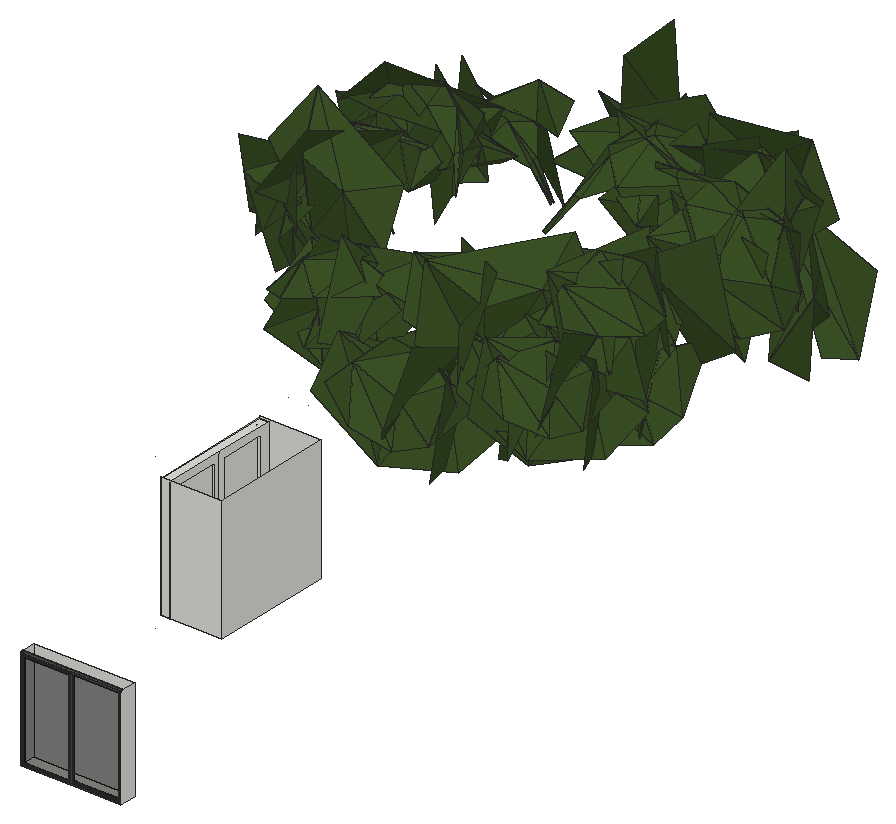
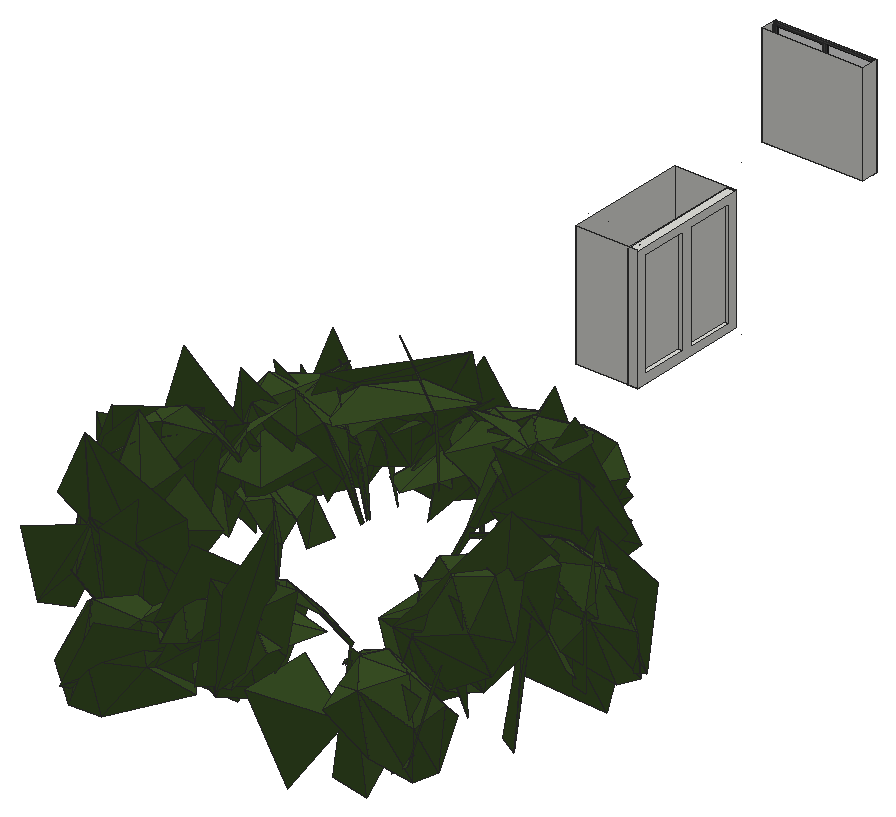
# SketchUp Ruby script. Lengths in inches.
U = 1.inch
M = Sketchup.active_model
def pt(a) = Geom::Point3d.new(a.map { |v| v * U })
def face(e, loops, mat)
  f = e.add_face(loops[0].map { |a| pt(a) })
  loops[1..].each { |l| e.add_face(l.map { |a| pt(a) }).erase! }
  f.material = f.back_material = mat if mat
  f
end
# faces: each face lists its corners as indices into pts; further lists are holes
def faces(e, pts, list, mat = nil) = list.each { |f| face(e, (f[0].is_a?(Array) ? f : [f]).map { |l| l.map { |i| pts[i] } }, mat) }
# xy, xz, yz: faces in a plane at the given z, y or x. An outline is a flat list of corners, or four numbers for a rectangle; further outlines are holes
def ring(l) = l.size == 4 ? [[l[0], l[1]], [l[2], l[1]], [l[2], l[3]], [l[0], l[3]]] : l.each_slice(2).to_a
def flat(e, list, mat, &to3) = list.each { |f| face(e, (f[0].is_a?(Array) ? f : [f]).map { |l| ring(l).map { |u, v| to3.(u, v) } }, mat) }
def xy(e, z, list, mat = nil) = flat(e, list, mat) { |x, y| [x, y, z] }
def xz(e, y, list, mat = nil) = flat(e, list, mat) { |x, z| [x, y, z] }
def yz(e, x, list, mat = nil) = flat(e, list, mat) { |y, z| [x, y, z] }
def lines(e, pts, list) = list.each { |a, b| e.add_line(pt(pts[a]), pt(pts[b])) }
# prism: a flat outline (further loops are holes) pulled along v
def prism(e, loops, v, mat = nil)
  f = face(e, loops, mat); d = Geom::Vector3d.new(v.map { |x| x * U })
  f.pushpull(f.normal.samedirection?(d) ? d.length : -d.length)
end
def box(e, o, s, mat = nil) = prism(e, [[o, [o[0] + s[0], o[1], o[2]], [o[0] + s[0], o[1] + s[1], o[2]], [o[0], o[1] + s[1], o[2]]]], [0, 0, s[2]], mat)
def at(x, y, z, deg = 0) = Geom::Transformation.translation(pt([x, y, z])) * Geom::Transformation.rotation(ORIGIN, Z_AXIS, deg.degrees)
def axes(o, x, y, z) = Geom::Transformation.new([*x, 0, *y, 0, *z, 0, *pt(o).to_a, 1])
def part(name) = M.definitions.add(name)
# library, detail: a bought-in or finely detailed component or shape, given as its bounding box
def library(name, o, s) = part(name).tap { |d| box(d.entities, o, s) }
def detail(e, o, s) = box(e.add_group.entities, o, s)
def put(e, d, t, mat = nil) = e.add_instance(d, t).tap { |i| i.material = mat if mat }
def group(e, t, mat = nil) = e.add_group.tap { |g| g.transformation = t; g.material = mat if mat }.entities
root = M.entities
M.materials.add("AM113_062_Tilia").color = [58, 81, 37]
M.materials.add("Glass_Tinted_Gray").color = [0, 0, 0]
M.materials["Glass_Tinted_Gray"].alpha = 0.125
M.materials.add("[0135_DarkGray]").color = [81, 81, 81]
M.materials.add("[Mirror 02]").color = [229, 229, 229]
M.materials.add("[Terrazzo Light Blue]").color = [196, 214, 227]
c1 = part("Window (2)")
xy(c1.entities,31.72,[[-0.78,88.6,2.72,128.1]])
xy(c1.entities,34.95,[[-0.78,91.53,0.84,106.59],[0.84,91.53,1.05,97.58],[1.05,91.53,1.42,106.59],[1.42,91.53,2.72,106.59],[0.84,97.58,1.05,98.18],
  [0.84,98.18,1.05,106.59]])
xy(c1.entities,35.27,[[-0.78,110.09,0.97,125.14],[1.05,110.09,2.72,125.14]])
xy(c1.entities,58.35,[[2.72,108.74,3.8,109.74]])
xy(c1.entities,77.8125,[[-0.78,110.09,2.72,125.14],[0.97,110.09,1.05,125.14]])
xy(c1.entities,77.93,[[-0.78,91.53,0.84,106.59],[1.05,91.53,1.42,106.59],[1.42,91.53,2.72,106.59]])
xy(c1.entities,80.72,[[-0.78,88.6,2.72,128.1]])
xz(c1.entities,88.6,[[-0.78,31.72,2.72,80.72]])
xz(c1.entities,91.53,[[-0.78,34.95,0.84,77.93],[1.05,34.95,1.42,77.93],[1.42,34.95,2.72,77.93]])
xz(c1.entities,106.59,[[-0.78,34.95,0.84,77.93],[0.84,34.95,1.05,77.93],[0.84,34.95,2.72,77.93]])
xz(c1.entities,108.74,[[3.8,54.35,4.22,54.6,4.22,59.47,2.72,59.97,2.72,58.35,3.8,58.35]])
xz(c1.entities,109.74,[[3.8,54.35,3.8,58.35,2.72,58.35,2.72,59.97,4.22,59.47,4.22,54.6]])
xz(c1.entities,110.09,[[-0.78,35.27,0.97,77.8125],[1.05,35.27,2.72,77.8125]])
xz(c1.entities,125.14,[[-0.78,35.27,0.97,77.8125],[0.97,35.27,1.05,80.72],[1.05,35.27,2.72,77.8125]])
xz(c1.entities,128.1,[[-0.78,31.72,2.72,80.72]])
yz(c1.entities,-0.78,[[[88.6,31.72,128.1,80.72],[91.53,34.95,106.59,77.93],[110.09,35.27,125.14,77.8125]]])
yz(c1.entities,0.84,[[91.53,34.95,106.59,77.93]])
yz(c1.entities,0.97,[[110.09,35.27,125.14,77.8125]])
yz(c1.entities,1.05,[[91.53,34.95,106.59,77.93],[110.09,35.27,125.14,77.8125]])
yz(c1.entities,1.42,[[91.53,34.95,106.59,77.93]])
yz(c1.entities,2.72,[[[88.6,31.72,108.35,80.72],[91.53,34.95,106.59,77.93]],[[108.35,31.72,128.1,80.72],[110.09,35.27,125.14,77.8125],[108.74,58.35,109.74,59.97]]])
yz(c1.entities,3.8,[[108.74,54.35,109.74,58.35]])
yz(c1.entities,4.22,[[108.74,54.6,109.74,59.47]])
p = [[4.22,108.74,54.6],[3.8,108.74,54.35],[3.8,109.74,54.35],[4.22,109.74,54.6],[2.72,109.74,59.97],[2.72,108.74,59.97],
  [4.22,108.74,59.47],[4.22,109.74,59.47],[-0.78,86.4,89.94],[-0.78,86.44,89.94],[15.22,130.69,89.94],[15.22,130.65,89.94],
  [-0.78,86.44,28.19],[-0.78,86.4,28.19],[7.72,130.69,89.94],[7.72,130.65,89.94]]
faces(c1.entities,p,[[0,1,2,3],[4,5,6,7]])
lines(c1.entities,p,[[8,9],[10,11],[12,13],[14,15]])
c2 = part("PENTEK_RP Fineline 50S_Sliding_DoorCase_E1")
box(c2.entities,[0,0,0],[1.51,3.66,99.27],"[0135_DarkGray]")
c3 = part("PENTEK_RP Fineline 50S_SlidingDooe_Case_E2")
box(c3.entities,[0,0,0],[96.25,3.66,1.51],"[0135_DarkGray]")
c4 = part("pentek_RP Fineline 50S_SlidingDoor_Case")
put(c4.entities,c2,at(97.76,0,0))
put(c4.entities,c3,at(1.51,0,0))
put(c4.entities,c2,at(0,0,0))
put(c4.entities,c3,at(1.51,0,97.76))
c5 = part("PENTEK_RP Fineline 50S_SlidingDoor_GlazingBead_2")
box(c5.entities,[0,0,0],[0.56,0.59,94.39],"[0135_DarkGray]")
c6 = part("PENTEK_RP Fineline 50S_SlidingDoor_Glass")
box(c6.entities,[0,0,0],[46.58,0.16,94.39],"Glass_Tinted_Gray")
c7 = part("PENTEK_RP Fineline 50S_SlidingDoor_GlazingBead")
box(c7.entities,[0,0,0],[45.47,0.59,0.56],"[0135_DarkGray]")
c8 = part("PENTEK_RP Fineline 50S_SlidingDoor_Leaf_E1")
xy(c8.entities,0,[[0,0,0.93,1.97],[0.93,1.57,1.49,1.97]],"[0135_DarkGray]")
xy(c8.entities,96.25,[[0,0,0.93,0,0.93,1.57,1.49,1.57,1.49,1.97,0,1.97]],"[0135_DarkGray]")
xz(c8.entities,0,[[0,0,0.93,96.25]],"[0135_DarkGray]")
xz(c8.entities,1.57,[[0.93,0,1.49,95.32],[0.93,95.32,1.49,96.25]],"[0135_DarkGray]")
xz(c8.entities,1.97,[[0,0,1.49,96.25]],"[0135_DarkGray]")
yz(c8.entities,0,[[0,0,1.97,96.25]],"[0135_DarkGray]")
yz(c8.entities,0.93,[[0,0,1.57,0.93],[0,0.93,1.57,95.32],[0,95.32,1.57,96.25]],"[0135_DarkGray]")
yz(c8.entities,1.49,[[1.57,0,1.97,95.32],[1.57,95.32,1.97,96.25]],"[0135_DarkGray]")
c9 = part("PENTEK_RP Fineline 50S_SlidingDoor_Leaf_E2")
xy(c9.entities,0,[[0,0,0,1.57,0.56,1.57,0.56,1.97,46.02,1.97,46.02,1.57,46.58,1.57,46.58,0]],"[0135_DarkGray]")
xy(c9.entities,0.93,[[0,0,46.58,1.57]],"[0135_DarkGray]")
xy(c9.entities,1.49,[[0.56,1.57,46.02,1.97]],"[0135_DarkGray]")
xz(c9.entities,0,[[0,0,46.58,0.93]],"[0135_DarkGray]")
xz(c9.entities,1.57,[[0,0,0.56,0.93],[46.02,0,46.58,0.93],[0.56,0.93,46.02,1.49]],"[0135_DarkGray]")
xz(c9.entities,1.97,[[0.56,0,46.02,1.49]],"[0135_DarkGray]")
yz(c9.entities,0,[[0,0,1.57,0.93]],"[0135_DarkGray]")
yz(c9.entities,0.56,[[1.57,0,1.97,0.93],[1.57,0.93,1.97,1.49]],"[0135_DarkGray]")
yz(c9.entities,46.02,[[1.57,0,1.97,0.93],[1.57,0.93,1.97,1.49]],"[0135_DarkGray]")
yz(c9.entities,46.58,[[0,0,1.57,0.93]],"[0135_DarkGray]")
c10 = part("PENTEK_RP Fineline S_SlidingDoor_Leaf1")
put(c10.entities,c5,at(0.93,0,0.93))
put(c10.entities,c5,at(46.96,0,0.93))
put(c10.entities,c6,at(1.49,1.42,0.93))
put(c10.entities,c7,at(1.49,0,0.93))
put(c10.entities,c6,at(1.49,0.59,0.93),"[Terrazzo Light Blue]")
put(c10.entities,c8,at(0,0,0))
put(c10.entities,c8,axes([48.44,0,0],[-1,0,0],[0,1,0],[0,0,1]))
put(c10.entities,c9,axes([0.93,0,96.25],[1,0,0],[0,1,0],[0,0,-1]))
put(c10.entities,c9,at(0.93,0,0))
put(c10.entities,c7,at(1.49,0,94.77))
c11 = part("PENTEK_RP Fineline 50S_SlidingDoor_Leaf2")
put(c11.entities,c6,at(1.49,1.42,0.93))
put(c11.entities,c7,at(1.49,0,94.77))
put(c11.entities,c5,at(46.96,0,0.93))
put(c11.entities,c6,at(1.49,0.59,0.93),"[Mirror 02]")
put(c11.entities,c5,at(0.93,0,0.93))
put(c11.entities,c8,at(0,0,0))
put(c11.entities,c8,axes([48.44,0,0],[-1,0,0],[0,1,0],[0,0,1]))
put(c11.entities,c7,at(1.49,0,0.93))
put(c11.entities,c9,axes([0.93,0,96.25],[1,0,0],[0,1,0],[0,0,-1]))
put(c11.entities,c9,at(0.93,0,0))
c12 = part("PENTEK - Slimmest Steel Sliding Door / Window\#1")
put(c12.entities,c4,at(0,-1.88,-0.09))
put(c12.entities,c10,at(1.51,-2.27,1.42))
put(c12.entities,c11,at(49.32,-0.3,1.42))
xy(root,336.96,[[418.81,422.72,490.37,567.03]])
xy(root,339.36,[[496.21,121.6875,613.65,141.4375]])
xz(root,141.4375,[[496.21,339.36,613.65,457.89]])
xz(root,422.72,[[418.81,336.96,490.37,481.27]])
xz(root,567.03,[[418.81,336.96,490.37,481.27]])
yz(root,490.37,[[422.72,336.96,567.03,481.27]])
yz(root,496.21,[[121.6875,339.36,141.4375,457.89]])
yz(root,613.65,[[121.6875,339.36,141.4375,457.89]])
p = [[441.03,1318.83,315.71],[374.57,1266.21,338.79],[410.33,1292.3,366.44],[464.57,1312.27,363.78],[476.36,1323.12,317.65],[227.63,1225.04,422.85],
  [207.89,1274.74,315.85],[135.38,1315.0625,337.2],[604.51,1143.52,417.32],[606.52,1132.49,335.45],[533.22,1166.68,316.28],[582.15,1192.12,368.28],
  [492.22,1222.92,340.89],[542.42,1231.33,389.63],[494.05,1268.36,398.42],[509.61,1301.62,344.19],[484.64,1326.68,337.1],[478.25,1295.32,318.57],
  [402.18,1251.8,365.35],[389.98,775.12,327.61],[447.13,822.39,320.07],[424.36,834.7,394.59],[471.65,860.97,354.9],[334.16,1166.82,415.15],
  [357.77,1225.61,320.1],[406.875,1283.29,364.77],[558.07,946.28,343.21],[540.23,970.85,320.5625],[514.18,1044.49,389.96],[97.48,1148.85,324.84],
  [125.97,1129.49,321.65],[142.76,1077.9,419.68],[262.51,1334.86,413.52],[218.8,1326.06,322.26],[203.26,1258.99,368.5],[447.77,803.34,428.45],
  [442.46,786.28,323.07],[426.5,862.23,323.94],[356.27,874.53,399.9],[128.03,1080.25,446.63],[86.76,1149.85,412.7],[437.29,913.49,424.69],
  [464.78,858.4,325.1875],[519.95,803.08,367.03],[608.48,1203.96,326.7],[577.22,1188.08,325.58],[521.47,1210.05,420.41],[485.66,953.18,370.83],
  [465.23,949.89,333.03],[526.24,936.19,326.52],[564.41,959.15,330.14],[530.41,1224.98,445.47],[613.15,1223.15,413.38],[309.1,819.54,422.23],
  [329.85,753.71,394.76],[380.76,799.52,408.42],[502.9,854.39,333.17],[540.33,916.03,329.79],[543.41,902.78,409.65],[561.26,954.88,369.74],
  [543.97,963.95,372.82],[573.51,990.87,347.42],[64.95,1009.39,435.27],[153.17,1068.44,482.16],[67.9,1049.2,332.93],[147.31,1072.73,355.1875],
  [452.77,1006.15,350.35],[466.24,836.61,462.78],[479.24,795.64,400.84],[520.45,849.67,418.12],[278.7,947.55,409.11],[265.15,869.36,333.42],
  [228.34,811.86,397.87],[389.27,1262.24,391.29],[448.08,1323.06,414.01],[119.7,1255.64,419.91],[73.95,975.25,437.49],[103.41,985.12,337.34],
  [169.32,980.3,389.87],[403.66,1231.72,348.02],[486.86,1261.4,389.11],[558.89,882.58,451],[562.27,860.92,346.91],[530.12,931.41,341],
  [455.54,930.67,411.53],[407.57,1207.09,440.2],[429.24,1241.74,377.59],[355.59,1260.08,341.24],[374.95,1261.49,424.31],[290.53,1278.1875,369.72],
  [319.55,1269.63,440.14],[513.37,838.62,349.09],[559.08,897.02,341.43],[530.8,906.71,413.42],[572.96,941.29,374.71],[518.65,1044.38,423.1],
  [541.84,961.25,428.94],[104.25,1038.67,343.52],[133.35,971.02,357.18],[118.71,989.55,432.95],[94,1040.9,430.01],[121.17,1104.63,467.66],
  [73.21,1102.1875,398.03],[516.83,1245.3,378.62],[126.73,1040.85,344.6],[159.33,978.85,366.98],[112.86,980.4,422.55],[78.85,1025.48,404.25],
  [69.41,1078.28,453.05],[62.41,1087.72,371.3125],[101.75,1251.73,347.14],[141.38,1175.32,359.86],[124.67,1213.99,392.62],[115.76,1271.09,395.66],
  [104.68,1287.05,351.76],[544.88,1017.89,399.71],[544.5,1066.22,387.94],[404.34,1238.19,384.97],[420.56,867.51,435.13],[456.39,806.95,414.03],
  [495.36,863.33,427.25],[104.04,1294.86,372.04],[132.27,1283.47,349.57],[162.55,1198.23,386.32],[455.45,1017.5,385.01],[231.01,1125.11,452.83],
  [175.01,1127.54,350.45],[119.73,1187.85,370.66],[424.95,1084.16,350.72],[444.2,1052.48,377.875],[444.11,1058.61,382.41],[423.89,1086.46,355.09],
  [447.05,1062.75,377.85],[427.01,1086.08,351.69],[166.625,1289.7,426.85],[133.91,1314.1,377.74],[59.77,1010.17,353.94],[80.93,984.08,369.2],
  [61.43,1013.52,404.26],[72.53,1067.11,433.74],[53.4,1052.84,368.66],[423.22,907.99,376.45],[321.53,965.23,355.26],[301.45,948.83,398.92],
  [307.53,952.08,400.95],[323.7,968.2,357.95],[371.51,1270.96,355.55],[369.36,1233.12,426.53],[382.18,1162.07,405.51],[426.26,1215.28,383.75],
  [319.26,1256.33,439.7],[306.85,1298.32,382.49],[311.99,949.18,396.875],[324.13,964.29,356.46],[145.625,937.05,407.37],[420.61,743.09,385.79],
  [403.99,765.4,358.24],[409.41,855.85,394.39],[181.4,1196.65,366.84],[47.53,1017.54,367.125],[80.77,1027.68,360.93],[139.61,998.33,449.09],
  [347.48,888.84,391.63],[327.78,909.84,361.97],[325.66,911.85,365.69],[325.25,908.46,362.48],[342.71,880.28,397.07],[344.85,886.94,398.42],
  [416.77,972.76,456.07],[478.14,944.07,363.48],[547.6,918.42,416.27],[274.47,839.93,363.8125],[343.32,839.48,391.68],[313.91,854.66,461.42],
  [213.92,899.01,451.29],[198.09,850.32,400.8],[256.85,849.4375,448.07],[434.47,1271.23,399],[371.78,1263.29,464.8],[426.38,750.04,366.35],
  [445.09,780.34,365.35],[417.32,769.98,408.27],[434.92,825.08,407.89],[441.87,866.59,375.05],[414.17,1184.43,385.54],[410.78,1151.13,365.68],
  [410.35,1149.02,370.19],[359.94,776.29,425.875],[385.09,739.13,383.06],[417.02,1184.89,392.6],[413.4,1150.14,366.7],[423.625,1187.02,390.93],
  [177.48,1196.72,404.39],[532.65,859.06,454.45],[162.07,941.07,416.47],[130.42,985.74,476.0625],[47,1001.33,455.01],[502.68,1056.83,367.57],
  [495.52,1044.96,400.97],[284.51,1219.8125,394.78],[85.3,1095.68,411.12],[148.9,964.22,433.6],[103.04,981.9,436.22],[444.24,942.37,401.65],
  [421.83,957.38,369.28],[419.16,959.01,372.7],[591.32,1092.38,480.73],[481.53,1087.52,509.95],[576.66,1077.39,369.4],[495.99,1099.81,385.01],
  [305.1,1166.72,409.37],[284.47,1147.6,373.08],[286.98,1149.55,369.61],[311.46,1168.29,406.34],[536.41,960.06,432.07],[419.64,955.49,369.73],
  [441.21,933.18,407.4375],[441.78,940.1875,408.41],[259.23,1279.27,425.01],[140.1875,1132.32,369.86],[117.9,1078.39,422.125],[127.2,1122.49,477.81],
  [138.81,1170.82,440.98],[194.82,1202.85,445.47],[162.35,1210.0625,375.77],[301.12,1169.65,404.77],[284.7,1151.13,370.5625],[136.28,1177.68,480.64],
  [508.18,1000.93,406.64],[396.31,865.26,371.11],[394.34,864.1,408.88],[151.38,1186.3,412.53],[105.02,1254.5,445.86],[481.28,1037.22,460.29],
  [554.07,1042.37,374.57],[620.73,1008.24,425.33],[514.55,977.19,389.66],[231.99,1195.9,399.33],[262.63,1187.13,375.49],[264.88,1186.07,379.7],
  [130.08,1151.4375,376.6],[98.59,1097.97,426.83],[140.47,1121.43,478.11],[166.77,1164.62,446.6],[238.72,1168.11,424.6875],[188.5,1207.375,384],
  [232.53,1198.42,406.58],[264.18,1189.46,376.55],[231.66,1205.39,405.57],[192.47,1308.53,405.88],[472.79,1030.03,407.04],[468.56,1211.1,379.65],
  [344.09,1281.55,478.4],[340.7,1310.04,378.85],[280.83,1262.56,380.15],[446.25,1214.8,403.67],[474.21,916.14,499.13],[512.04,890.48,440.52],
  [512.19,957.86,379.7],[520.03,956.09,467.22],[515.56,1014.11,464.52],[515.625,1029.8125,385.3],[363.64,930.61,488.5625],[393.16,888.65,379.81],
  [443.67,825.43,411.66],[311.8,1181.32,415.01],[547.53,816.32,411.41],[527.73,833.38,381.23],[511.63,924.01,410.69],[260.99,828.87,382.35],
  [331.24,819.07,411.32],[311.57,867.58,457.24],[229.76,941.49,402.23],[195.96,877.6875,399.24],[256.87,878.47,441.87],[270.51,1292.74,430.41],
  [331.97,770.47,397.9],[489.47,1042.6,484.82],[537.02,1028.03,417.23],[551.4,1104.72,383.21],[550.49,1084.18,466.64],[558,1138.92,484.9],
  [563.22,1173.42,416.76],[548.11,1036.85,477.79],[556.41,1037.58,395.36],[531.52,1115.45,383.86],[573.91,1091.92,445.94],[568.84,1144.55,477.41],
  [536.51,1180.27,424.27],[475.17,1281.89,485.09],[487.7,1255.23,384.14],[428.76,1209.87,412.77],[422.34,1227.64,408.29],[510.71,1071.02,429.7],
  [420.69,862.05,423.64],[426.82,780.96,461.36],[497.89,929.43,385.97],[494.49,929.26,423.6],[542.58,900.17,428.06],[541.8,940.93,392.56],
  [509.63,1248.625,450.93],[398.83,1296.59,419.6875],[380.47,1279.51,389.0625],[306.55,1234.6,434.43],[387.18,848.2,509.98],[401.15,815.75,440.45],
  [430.62,881.46,389.22],[443.92,864.14,472.72],[469.66,916.1875,478.3],[470.95,940.38,402.74],[357.53,1186.72,391.57],[411.4375,1208.73,389.5],
  [400.98,1222.35,429.31],[415.43,1269.91,399.09],[552.52,823.66,391.86],[564.19,857.26,389.67],[537.43,842.625,431.58],[164.82,1044.58,475.43],
  [522.74,1217.73,404.87],[453.67,1242.86,389.97],[457.25,1239.625,471.39],[409.79,1256.52,424.26],[335.43,829.3,391.01],[347.7,846.8,416.85],
  [371.26,858.33,426.9375],[342.52,1182.73,422.93],[375.64,853.95,444.12],[479.35,836.74,445.16],[513.91,804.52,406.84],[152.03,1231.9,424.0625],
  [602.43,1124.55,493.04],[582.09,1148.22,392.96],[525.3,1181.29,446.24],[258.94,919.7,393.28],[209.53,887.84,401.87],[223.3,883.5,444.23],
  [273.625,931.87,421.96],[509.44,1199.9,399.75],[439.87,1218.46,393.67],[457.26,1250.32,460.71],[399.6875,1241.68,429.08],[533.93,1000.77,508.45],
  [558.98,990.48,406.39],[498.17,1037.78,394.26],[425.89,997.32,447.3125],[212.85,1142.6,420.2],[194.09,1194.37,395.68],[179.34,1194.75,437.07],
  [133.125,1203.58,400.46],[292.46,845.16,504.67],[299.77,800.7,413.8],[350.08,858.32,396.82],[303.82,937.61,411.17],[293.42,927.56,445.71],
  [314.74,910.03,445.95],[423.01,923.79,462.16],[485.34,888.81,448.61],[526.98,947.81,397.53],[490.74,955.71,470.84],[502.33,1011.4,465.5],
  [539.62,1021.09,400.7],[261.05,855.36,488.41],[205.89,1046.26,493.72],[154.49,1005.75,398.43],[113.93,940.78,444.78],[387.67,1005.2,398.5],
  [412.74,993.1,440.15],[409.78,999.45,441.31],[385.24,1007.86,401.35],[411.63,1002.99,435.21],[388.72,1007.92,398.55],[285.51,1337.95,510.02],
  [311.57,1231.49,527.85],[297.9,1332.25,398.6],[291.69,1249.47,407.36],[386.8,1302.83,405.82],[192.78,1211.12,427.48],[515.01,1244.32,466.3125],
  [545.64,1214.17,530.3],[576.91,1214,457.61],[209.78,1232.27,422.88],[216.36,1254.6,399.94],[98.49,1179.7,416.82],[227.15,944.43,400.56],
  [271,933.08,438.27],[217.77,940.07,481.23],[159.08,967.8125,407.31],[526.76,1064.21,437.03],[553.48,1050.48,462.32],[583.28,1060.94,402.95],
  [602.84,1101.04,401.26],[594.89,1091.74,449.28],[598.24,1131.625,424.04],[472.44,919.2,440.64],[344.35,884.9375,487],[378.27,826.33,454.53],
  [439.58,863.18,401.88],[217.76,829.26,428.83],[419.11,877.71,483.22],[457.1,920.25,482.08],[488.22,919.05,410.98],[372.27,907.37,434.73],
  [491.73,971.87,452.41],[529.37,1038.09,432.02],[99.1,1017.88,460.46],[325.34,1194.44,445.05],[307.95,1215.07,440.91],[445.51,881.68,404.86],
  [454.66,823.86,416],[452.46,902.39,430.02],[509.54,1222.34,490.53],[526.82,1158.25,536.05],[573.35,1195.82,483.78],[252.34,1226.74,430.95],
  [380.99,1276.42,441.3125],[353,1304.77,417.61],[161.33,951.24,492.76],[138.53,1002.19,537.28],[99.125,979.55,478.33],[186.7,971.18,464.8125],
  [398.49,821.63,431.13],[298.91,1225.18,407.97],[326.13,1266.14,455.88],[280.96,1260.99,434.37],[519.9375,933.62,440.07],[502.54,957.18,454.9],
  [135.8,1076.71,442.48],[367.15,839.68,454.18],[541.86,857.36,484.25],[454.82,867.67,511.41],[455.06,1167.68,513.36],[306.93,859.58,476.58],
  [350.56,869.29,450.07],[325.18,896.14,415.41],[522.01,967.56,505.81],[147.18,958.95,480.15],[567,1200.09,475.76],[94.41,1150.57,441.45],
  [124.04,1181.42,454.05],[302.43,1234.07,467.12],[378,1266.59,495.13],[215.53,1135.73,456.17],[278.88,888.9,471.28],[114.23,1062.09,487.12],
  [347.64,1232.28,458.3],[506.78,889.62,449.28],[574.84,1135.77,490.17],[546.89,1176.17,493.33],[550.34,1204.76,483.61],[392.67,1202.37,476],
  [166.18,1054.32,497.88],[273.02,1243.45,473.52],[580.85,1025.4375,525.26],[101.38,1074.77,487.14],[252.875,803.79,442.32],[405.97,1239.24,498.94],
  [229.48,1096.13,458.97],[247.84,1066.83,433.59],[246.08,1068.46,429.2],[228.33,1101.52,453.48],[479.64,1059.63,485.6875],[226.39,1091.4,456.05],
  [244.36,1066.61,430.96],[466.08,1017.83,431.44],[458.96,1013.5,467.77],[514,1010.16,482.44],[497.91,1048.07,447.74],[495.09,1077.05,468.6875],
  [159.6875,1008.5,437.61],[137.08,1060.18,473.625],[442.71,993.16,479.59],[144,1010.63,469.52],[457.33,1067.37,439.28],[165.9,1151.64,485.51],
  [441.32,950.02,437.99],[475.55,902.72,450.35],[487.51,923.61,484.66],[434.61,969.75,464.55],[272.94,959.61,499.74],[133.64,1084.04,488.14],
  [130.87,1132.36,490.29],[254.0625,836.76,469.59],[287.12,810.29,451.73],[355.67,894.67,483.27],[174.43,942.02,528.64],[150.15,1085.0625,529.3],
  [485.64,1114.26,510.56],[557.54,985.22,448.91],[537.17,914.12,454.17],[563.2,950.0625,448.13],[536.58,956.93,484.14],[556.05,1100.99,503.125],
  [464.28,969.77,513.19],[202.53,1125.36,483.52],[445.26,993.68,474.09],[180.97,1108.9,485.63],[170.78,1092.88,457.49],[137.21,1034.375,485.42],
  [500.17,1086.39,503.9],[485.6,982.65,495.34],[181.9375,1049.26,479.15],[215.625,1062.72,470.87],[216.27,1064.22,475.73],[214.85,1065.53,470.875],
  [173.77,1056.12,479.16],[178.24,1052.29,484.22],[508.875,1187.16,522.08],[546.82,1172.46,540.18],[513.27,1146.04,484.31],[522.05,1130.72,514.58],
  [433.2,1126.25,500.5],[471.55,1109.46,510.89],[469.49,1114.3,516.99],[432.29,1127.375,505.625],[468.57,1119.57,512.99],[434.1,1128.95,501.33],
  [513.125,1105.43,522.98]]
faces(root,p,[[0,1,2],[3,0,2],[4,0,3],[5,6,7],[8,9,10],[10,11,8],[10,12,13],[13,11,10],
  [4,3,14],[14,15,4],[16,17,18],[19,20,21],[20,22,21],[23,24,25],[26,27,28],[29,30,31],
  [32,33,34],[35,36,37],[35,37,38],[31,39,29],[39,40,29],[41,42,43],[44,45,46],[47,48,49],
  [47,49,50],[46,51,44],[51,52,44],[53,54,19],[19,55,53],[21,55,19],[56,57,58],[57,59,58],
  [50,60,47],[50,61,60],[62,63,64],[63,65,64],[66,48,47],[67,68,56],[56,69,67],[58,69,56],
  [70,71,72],[18,73,16],[73,74,16],[75,5,7],[76,77,78],[2,1,79],[12,80,13],[81,82,83],
  [81,83,84],[85,86,87],[87,88,85],[87,89,90],[90,88,87],[91,92,93],[92,94,93],[28,95,26],
  [95,96,26],[97,98,99],[99,100,97],[101,102,97],[97,100,101],[14,103,15],[104,105,106],[106,107,104],
  [104,107,108],[108,109,104],[110,111,112],[113,110,112],[114,110,113],[60,61,115],[61,116,115],[79,117,2],
  [118,119,91],[91,120,118],[93,120,91],[121,122,123],[47,124,66],[125,126,127],[128,129,130],[130,131,128],
  [132,133,131],[114,113,134],[134,135,114],[136,137,138],[139,140,136],[136,138,139],[21,22,141],[131,130,132],
  [142,143,144],[144,145,142],[146,147,148],[148,149,146],[150,147,146],[146,151,150],[152,153,145],[98,154,99],
  [145,144,152],[155,156,157],[112,111,158],[159,160,161],[162,163,164],[165,166,167],[167,164,165],[168,169,170],
  [171,172,173],[174,175,171],[171,176,174],[173,176,171],[14,3,177],[177,3,2],[178,23,25],[179,180,181],
  [181,180,182],[180,183,182],[164,167,162],[184,185,186],[187,188,179],[179,181,187],[177,2,117],[189,186,190],
  [190,191,189],[158,192,112],[193,41,43],[105,194,106],[195,196,159],[161,195,159],[197,198,115],[115,116,197],
  [8,11,13],[32,34,199],[139,200,140],[137,201,202],[138,137,202],[203,204,205],[206,207,208],[207,209,208],
  [210,211,212],[212,213,210],[58,59,214],[215,216,217],[217,205,215],[89,218,90],[219,220,221],[221,222,219],
  [219,222,223],[223,224,219],[186,189,184],[225,226,211],[227,125,127],[124,47,228],[47,60,228],[229,230,182],
  [182,183,229],[123,231,121],[231,232,121],[205,217,203],[228,60,115],[211,210,225],[233,234,235],[93,94,236],
  [237,238,239],[21,141,53],[240,241,242],[242,243,240],[244,245,240],[240,243,244],[246,239,247],[247,248,246],
  [134,249,135],[129,124,250],[132,130,250],[250,130,129],[250,198,132],[251,103,14],[252,253,254],[14,255,251],
  [256,257,258],[258,259,256],[260,259,258],[258,261,260],[239,246,237],[262,263,264],[252,254,265],[266,267,268],
  [269,270,271],[272,273,269],[269,274,272],[271,274,269],[151,275,150],[187,276,188],[277,278,279],[279,280,277],
  [281,280,279],[279,282,281],[283,284,285],[285,286,283],[287,286,285],[285,288,287],[289,290,291],[228,250,124],
  [292,117,184],[177,117,292],[261,293,260],[184,189,292],[157,294,155],[294,295,155],[296,297,298],[298,299,296],
  [13,80,300],[301,302,303],[304,305,306],[306,307,304],[308,307,306],[306,309,308],[310,311,312],[312,311,313],
  [13,300,8],[314,315,316],[316,315,298],[315,299,298],[93,236,118],[76,78,317],[318,319,320],[319,321,320],
  [292,189,191],[191,255,292],[322,276,187],[187,323,322],[162,167,324],[324,230,162],[312,325,310],[172,326,173],
  [327,328,314],[314,316,327],[329,112,192],[329,113,112],[330,331,332],[333,334,335],[335,336,333],[337,338,339],
  [338,340,339],[341,342,343],[341,343,344],[53,55,21],[345,346,347],[347,346,348],[134,113,329],[349,350,351],
  [349,351,352],[353,354,152],[152,144,353],[166,323,324],[324,167,166],[355,356,357],[357,358,355],[359,358,357],
  [357,360,359],[361,70,72],[362,363,364],[255,14,177],[365,366,367],[367,368,365],[369,370,368],[371,372,373],
  [372,374,373],[143,336,353],[353,144,143],[177,292,255],[312,313,375],[376,192,237],[237,246,376],[228,115,198],
  [339,377,337],[378,379,337],[337,377,378],[134,380,381],[381,249,134],[347,348,382],[383,384,385],[386,383,385],
  [360,387,359],[228,198,250],[368,367,369],[388,389,390],[390,391,388],[390,392,391],[203,217,393],[393,297,203],
  [394,395,396],[335,334,397],[396,398,394],[399,398,396],[396,400,399],[271,401,272],[272,274,271],[309,402,308],
  [388,403,389],[108,107,106],[404,138,202],[139,138,404],[329,192,376],[225,210,405],[405,406,225],[407,408,327],
  [327,409,407],[318,410,411],[411,412,318],[320,410,318],[150,413,148],[148,147,150],[376,246,248],[248,380,376],
  [375,414,312],[375,415,414],[405,210,213],[213,325,405],[327,408,328],[385,416,386],[386,416,417],[417,418,386],
  [216,409,393],[393,217,216],[99,154,419],[420,181,182],[420,182,230],[421,406,422],[422,423,421],[187,181,420],
  [420,230,324],[58,214,67],[67,69,58],[268,424,266],[400,425,399],[426,200,139],[270,427,271],[424,428,266],
  [429,262,264],[289,291,430],[118,120,93],[431,432,433],[433,354,431],[434,168,170],[106,194,435],[323,187,420],
  [420,324,323],[282,436,281],[382,437,438],[382,438,347],[415,423,422],[414,415,422],[303,439,301],[439,440,301],
  [347,441,345],[336,335,442],[442,353,336],[220,443,221],[106,435,108],[444,405,325],[325,312,444],[329,376,380],
  [380,134,329],[445,297,393],[445,298,297],[391,392,446],[392,447,446],[288,448,287],[320,321,449],[85,88,90],
  [242,450,244],[244,243,242],[90,218,451],[452,233,235],[241,453,242],[445,316,298],[335,397,454],[339,340,455],
  [456,457,458],[458,459,456],[312,414,444],[260,293,460],[409,327,445],[445,393,409],[101,100,99],[150,275,413],
  [461,462,457],[463,464,465],[465,466,463],[327,316,445],[467,403,388],[99,419,101],[202,201,468],[457,456,461],
  [469,139,404],[139,469,426],[271,427,401],[369,367,470],[470,464,369],[404,202,471],[468,471,202],[359,387,472],
  [441,347,473],[347,438,473],[474,475,476],[476,477,474],[385,384,478],[359,472,355],[90,451,85],[366,477,470],
  [470,367,366],[444,406,405],[444,422,406],[223,222,221],[444,414,422],[437,479,480],[438,437,480],[454,481,335],
  [454,482,481],[173,326,483],[335,481,442],[484,362,364],[221,485,223],[442,354,353],[442,431,354],[283,286,287],
  [330,332,486],[487,466,465],[174,176,173],[476,488,489],[489,490,476],[489,487,490],[490,487,465],[388,391,491],
  [491,391,446],[482,432,431],[476,475,488],[173,483,174],[481,482,431],[308,402,492],[493,456,459],[459,441,493],
  [473,438,480],[399,425,494],[493,495,461],[461,456,493],[473,493,441],[480,479,496],[496,495,480],[404,471,497],
  [404,497,469],[339,455,378],[378,377,339],[355,358,359],[388,498,467],[498,388,491],[260,460,256],[256,259,260],
  [477,476,499],[499,470,477],[277,280,281],[499,464,470],[499,465,464],[497,471,500],[442,481,431],[500,501,502],
  [503,504,505],[505,502,503],[320,449,411],[411,410,320],[304,307,308],[504,469,497],[399,494,394],[502,505,500],
  [281,436,506],[287,507,283],[287,448,507],[221,443,485],[242,453,450],[308,492,304],[500,505,497],[497,505,504],
  [385,478,417],[417,416,385],[394,398,399],[499,490,465],[473,495,493],[476,490,499],[508,509,446],[446,447,508],
  [281,506,277],[473,480,495],[491,446,509],[510,511,512],[512,513,510],[514,515,513],[491,516,498],[491,509,516],
  [511,498,516],[513,512,514],[516,512,511],[516,509,514],[514,512,516]],"AM113_062_Tilia")
put(root,c1,axes([421.25,100.07,244.3],[3.1248,0,0],[0,3.64173,0],[0,0,2.91389]))
put(root,c12,axes([496.21,123.56,339.47],[1.18298,0,0],[0,1,0],[0,0,1.194]))
